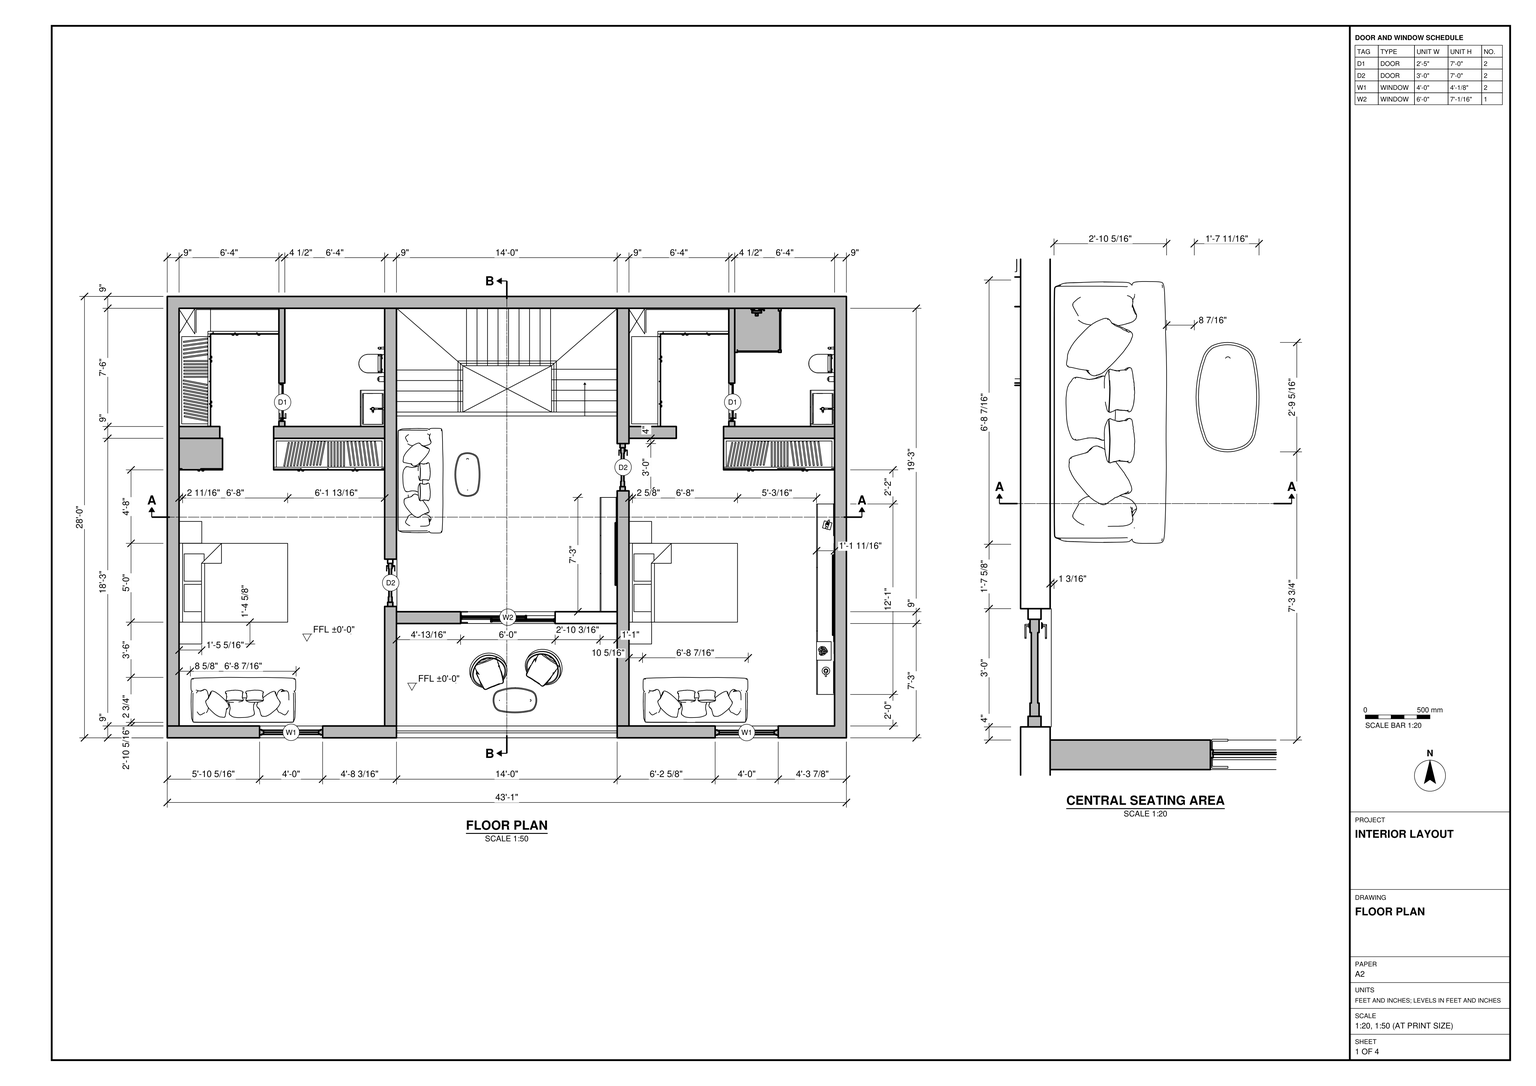
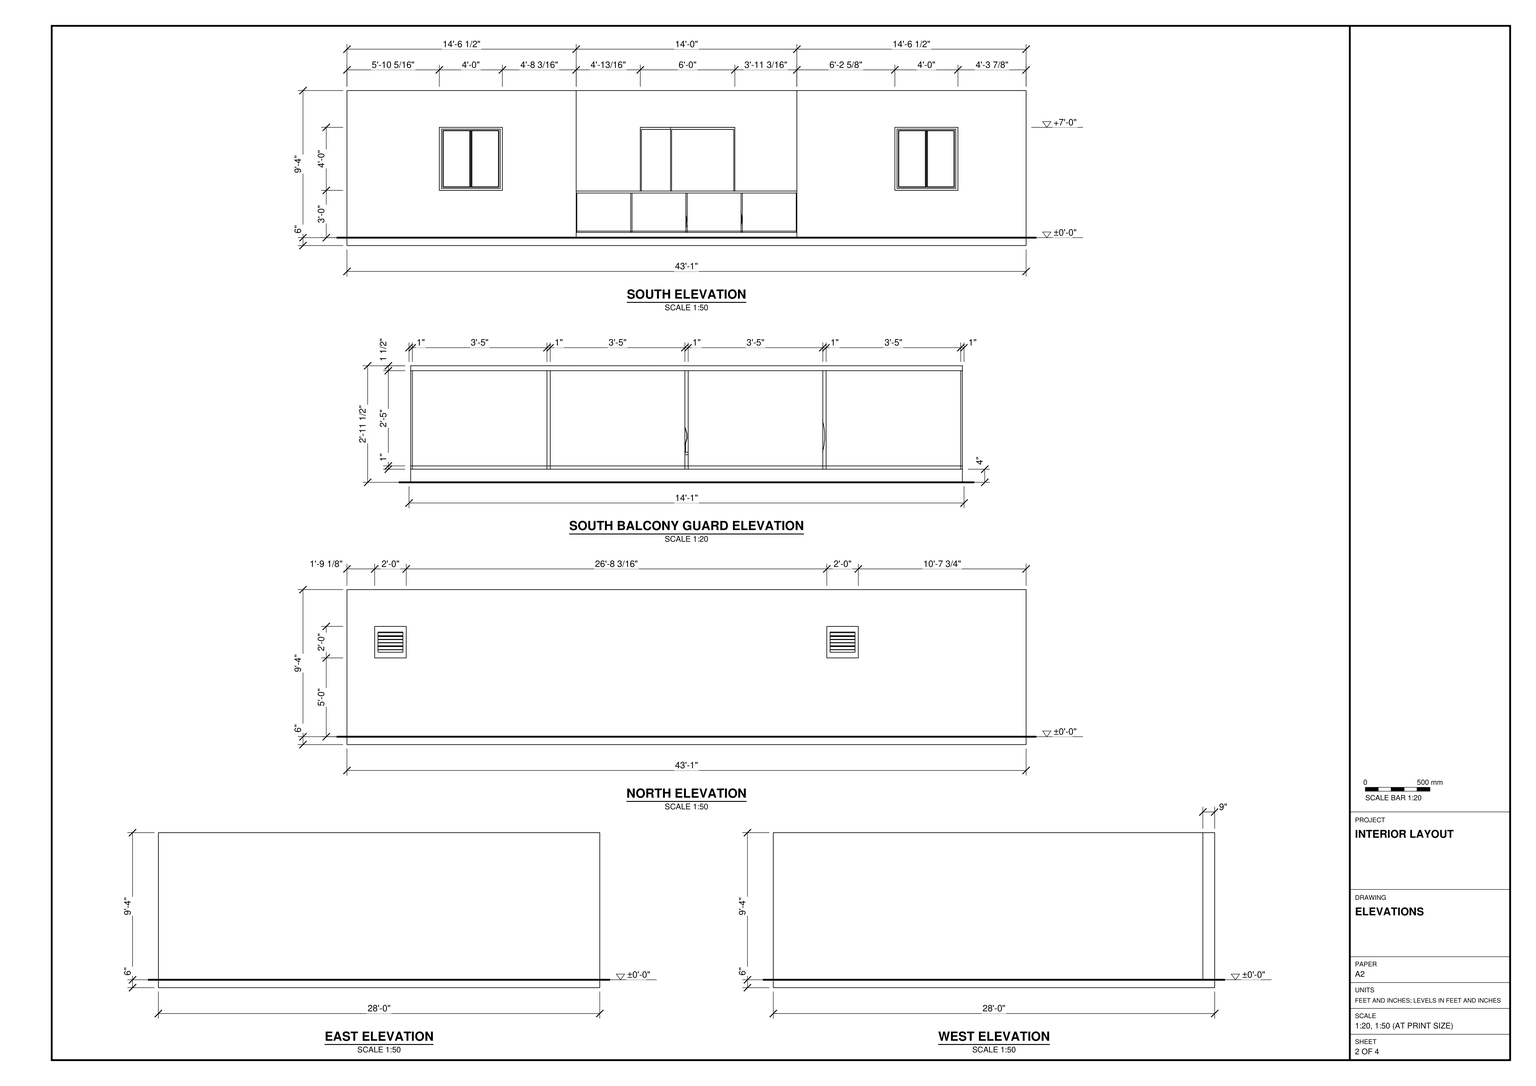
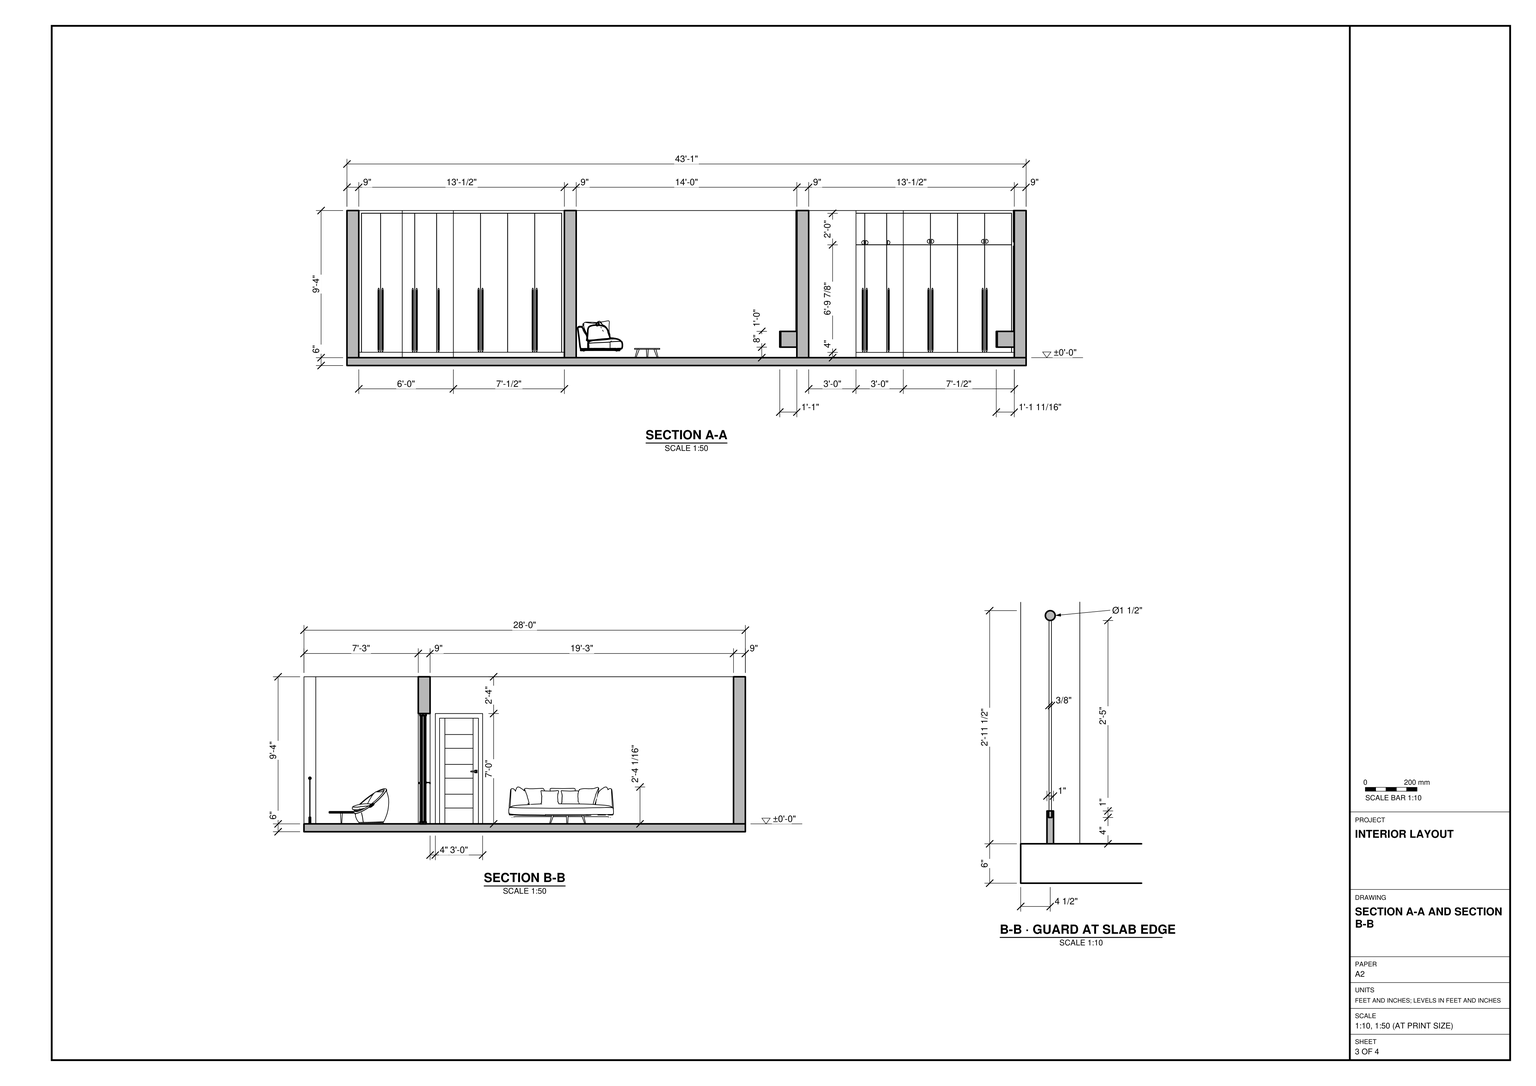
Build the single-storey interior in SketchUp from task_files/diagram_01.pdf. Work in feet and inches. Set the finished floor level to ±0'-0". The model measures 43'-1" east to west, 28'-0" north to south and 9'-10" from the underside of the slab to the top of the walls. Model the 6" floor slab, the 9" perimeter and main dividing walls, and the 4 1/2" partitions shown on the plan.

Lay out the two bedroom suites on either side of the 14'-0" central bay. In each suite, place the bed and sofa as drawn, fit the wardrobe and storage units along the indicated wall runs, and model the dressing area and adjoining bathroom with its fixtures. In the central bay, model the stair at the north end and the sitting area with the sofa, low table and facing wall unit. Recess the balcony between the bedrooms at the south end. Include its pair of chairs, table and panelled guard at the slab edge.

Fit the doors and window units to the scheduled openings. Use the elevations to locate the bedroom windows, the wider glazed opening facing the balcony and the louvred openings on the north wall. Keep shell elements and each furniture or joinery piece in separate groups or components, and use components for repeated parts. Decor and loose items may be any suitable library components, for example from 3D Warehouse. Save one SketchUp model as output_files/two_bedroom_suites_with_central_lounge_and_balcony.skp.

# SketchUp Ruby script. Lengths in inches.
U = 1.inch
M = Sketchup.active_model
def pt(a) = Geom::Point3d.new(a.map { |v| v * U })
def face(e, loops, mat)
  f = e.add_face(loops[0].map { |a| pt(a) })
  loops[1..].each { |l| e.add_face(l.map { |a| pt(a) }).erase! }
  f.material = f.back_material = mat if mat
  f
end
# faces: each face lists its corners as indices into pts; further lists are holes
def faces(e, pts, list, mat = nil) = list.each { |f| face(e, (f[0].is_a?(Array) ? f : [f]).map { |l| l.map { |i| pts[i] } }, mat) }
# xy, xz, yz: faces in a plane at the given z, y or x. An outline is a flat list of corners, or four numbers for a rectangle; further outlines are holes
def ring(l) = l.size == 4 ? [[l[0], l[1]], [l[2], l[1]], [l[2], l[3]], [l[0], l[3]]] : l.each_slice(2).to_a
def flat(e, list, mat, &to3) = list.each { |f| face(e, (f[0].is_a?(Array) ? f : [f]).map { |l| ring(l).map { |u, v| to3.(u, v) } }, mat) }
def xy(e, z, list, mat = nil) = flat(e, list, mat) { |x, y| [x, y, z] }
def xz(e, y, list, mat = nil) = flat(e, list, mat) { |x, z| [x, y, z] }
def yz(e, x, list, mat = nil) = flat(e, list, mat) { |y, z| [x, y, z] }
def lines(e, pts, list) = list.each { |a, b| e.add_line(pt(pts[a]), pt(pts[b])) }
# prism: a flat outline (further loops are holes) pulled along v
def prism(e, loops, v, mat = nil)
  f = face(e, loops, mat); d = Geom::Vector3d.new(v.map { |x| x * U })
  f.pushpull(f.normal.samedirection?(d) ? d.length : -d.length)
end
def box(e, o, s, mat = nil) = prism(e, [[o, [o[0] + s[0], o[1], o[2]], [o[0] + s[0], o[1] + s[1], o[2]], [o[0], o[1] + s[1], o[2]]]], [0, 0, s[2]], mat)
def at(x, y, z, deg = 0) = Geom::Transformation.translation(pt([x, y, z])) * Geom::Transformation.rotation(ORIGIN, Z_AXIS, deg.degrees)
def axes(o, x, y, z) = Geom::Transformation.new([*x, 0, *y, 0, *z, 0, *pt(o).to_a, 1])
def part(name) = M.definitions.add(name)
# library, detail: a bought-in or finely detailed component or shape, given as its bounding box
def library(name, o, s) = part(name).tap { |d| box(d.entities, o, s) }
def detail(e, o, s) = box(e.add_group.entities, o, s)
def put(e, d, t, mat = nil) = e.add_instance(d, t).tap { |i| i.material = mat if mat }
def group(e, t, mat = nil) = e.add_group.tap { |g| g.transformation = t; g.material = mat if mat }.entities
root = M.entities
M.materials.add("0207 AP 9584 Fervent Fuchsia-N").color = [176, 89, 135]
M.materials.add("0210 AP 9427 DELICATE PINK").color = [242, 226, 232]
M.materials.add("Glass Railing Color").color = [198, 198, 198]
M.materials.add("Railing Glass").color = [63, 150, 137]
M.materials["Railing Glass"].alpha = 0.13
M.materials.add("TEAKcrown-cut").color = [186, 122, 55]
M.materials.add("[Color M09]").color = [0, 0, 0]
M.materials.add("[Translucent Glass Gray]").color = [128, 128, 128]
M.materials["[Translucent Glass Gray]"].alpha = 0.5
M.materials.add("[Translucent_Glass_Gray]3").color = [255, 255, 255]
M.materials["[Translucent_Glass_Gray]3"].alpha = 0.5
M.materials.add("[Wood Floor]").color = [155, 105, 61]
M.materials.add("[Wood Veneer 02]").color = [190, 128, 91]
M.materials.add("dssd").color = [209, 209, 208]
c1 = library("Sliding windows",[317.26,-0.89,0.35],[175.04,8.85,122.84])
c2 = part("window full")
xy(c2.entities,0,[[0,0,14.17,66.54]])
xy(c2.entities,2.26,[[12.2,2.26,14.17,64.28]],"[Wood Floor]")
xy(c2.entities,2.36,[[0,2.36,1.97,64.17]],"[Wood Floor]")
xy(c2.entities,3.74,[[11.42,3.74,12.2,32.875],[11.42,33.66,12.2,62.79]],"[Wood Floor]")
xy(c2.entities,3.9375,[[1.97,3.9375,2.76,32.77],[1.97,33.76,2.76,62.6]],"[Wood Floor]")
xy(c2.entities,4.18,[[2.76,4.18,7.09,32.09],[7.09,4.18,11.42,32.09],[2.76,34.45,7.09,62.35],[7.09,34.45,11.42,62.35]],"[Wood Floor]")
xy(c2.entities,69.83,[[2.76,4.18,7.09,32.09],[7.09,32.09,11.42,34.45],[2.76,34.45,7.09,62.35]])
xy(c2.entities,69.83,[[7.09,4.18,11.42,32.09],[7.09,34.45,11.42,62.35]],"[Wood Floor]")
xy(c2.entities,70.08,[[1.97,3.9375,2.76,32.77],[1.97,33.76,2.76,62.6]])
xy(c2.entities,70.27,[[11.42,32.875,12.2,33.66]])
xy(c2.entities,70.27,[[11.42,3.74,12.2,32.875],[11.42,33.66,12.2,62.79]],"[Wood Floor]")
xy(c2.entities,71.65,[[0,2.36,1.97,64.17]])
xy(c2.entities,71.76,[[12.2,2.26,14.17,64.28]],"[Wood Floor]")
xy(c2.entities,74.02,[[0,0,14.17,66.54]],"[Wood Floor]")
xz(c2.entities,0,[[0,0,14.17,74.02]],"[Wood Floor]")
xz(c2.entities,2.26,[[12.2,2.26,14.17,71.76]],"[Wood Floor]")
xz(c2.entities,2.36,[[0,2.36,1.97,71.65]],"[Wood Floor]")
xz(c2.entities,3.74,[[11.42,3.74,12.2,70.27]],"[Wood Floor]")
xz(c2.entities,3.9375,[[1.97,3.9375,2.76,70.08]],"[Wood Floor]")
xz(c2.entities,4.18,[[2.76,4.18,7.09,69.83],[7.09,4.18,11.42,69.83]],"[Wood Floor]")
xz(c2.entities,32.09,[[2.76,4.18,11.42,69.83]],"[Wood Floor]")
xz(c2.entities,32.77,[[1.97,3.9375,2.76,70.08]],"[Wood Floor]")
xz(c2.entities,32.875,[[11.42,3.74,12.2,70.27]],"[Wood Floor]")
xz(c2.entities,33.66,[[11.42,3.74,12.2,47.88],[11.42,47.88,12.2,70.27]],"[Wood Floor]")
xz(c2.entities,33.76,[[1.97,3.9375,2.76,70.08]],"[Wood Floor]")
xz(c2.entities,34.45,[[2.76,4.18,11.42,69.83]],"[Wood Floor]")
xz(c2.entities,62.35,[[2.76,4.18,7.09,69.83],[7.09,4.18,11.42,69.83]],"[Wood Floor]")
xz(c2.entities,62.6,[[1.97,3.9375,2.76,70.08]],"[Wood Floor]")
xz(c2.entities,62.79,[[11.42,3.74,12.2,70.27]],"[Wood Floor]")
xz(c2.entities,64.17,[[0,2.36,1.97,71.65]],"[Wood Floor]")
xz(c2.entities,64.28,[[12.2,2.26,14.17,71.76]],"[Wood Floor]")
xz(c2.entities,66.54,[[0,0,14.17,74.02]],"[Wood Floor]")
yz(c2.entities,0,[[[0,0,66.54,74.02],[2.36,2.36,64.17,71.65]]],"[Wood Floor]")
yz(c2.entities,1.97,[[[2.36,2.36,64.17,71.65],[33.76,3.9375,62.6,70.08],[3.9375,3.9375,32.77,70.08]]],"[Wood Floor]")
yz(c2.entities,2.76,[[32.77,3.9375,33.76,4.18],[32.77,4.18,33.76,69.83],[32.77,69.83,33.76,70.08]])
yz(c2.entities,2.76,[[[3.9375,3.9375,32.77,70.08],[4.18,4.18,32.09,69.83]],[[33.76,3.9375,62.6,70.08],[34.45,4.18,62.35,69.83]]],"[Wood Floor]")
yz(c2.entities,7.09,[[4.18,4.18,62.35,69.83]],"[Translucent Glass Gray]")
yz(c2.entities,11.42,[[32.875,69.83,33.66,70.27]])
yz(c2.entities,11.42,[[[3.74,3.74,32.875,70.27],[4.18,4.18,32.09,69.83]],[[33.66,3.74,62.79,70.27],[34.45,4.18,62.35,69.83]]],"[Wood Floor]")
yz(c2.entities,12.2,[[[2.26,2.26,64.28,71.76],[33.66,3.74,62.79,70.27],[3.74,3.74,32.875,70.27]]],"[Wood Floor]")
yz(c2.entities,14.17,[[[0,0,66.54,74.02],[2.26,2.26,64.28,71.76]]],"[Wood Floor]")
p = [[11.42,32.875,70.27],[11.42,32.875,70.28]]
lines(c2.entities,p,[[0,1]])
c3 = part("Component\#10")
box(c3.entities,[0,0,0],[19,0.25,3.7],"[Translucent_Glass_Gray]3")
c4 = part("Ventilation_window")
g1 = group(c4.entities,at(-76.91,6.38,0),"TEAKcrown-cut")
xy(g1,-1.7,[[0,0,24,3]])
xy(g1,2.5,[[2.5,0,21.5,3]])
xy(g1,17.5,[[2.5,0,21.5,3]])
xy(g1,21.7,[[0,0,24,3]])
xz(g1,0,[[[0,-1.7,24,21.7],[2.5,2.5,21.5,17.5]]],"TEAKcrown-cut")
xz(g1,3,[[[0,-1.7,24,21.7],[2.5,2.5,21.5,17.5]]])
yz(g1,0,[[0,-1.7,3,21.7]])
yz(g1,2.5,[[0,2.5,3,2.5,3,4.31,0,6.48],[3,4.31,3,17.5,0,17.5,0,6.48]])
yz(g1,21.5,[[0,2.5,3,17.5]])
yz(g1,24,[[0,-1.7,3,21.7]])
put(g1,c3,axes([2.5,3.14,11.94],[1,0,0],[0,0.58779,0.80902],[0,-0.80902,0.58779]))
put(g1,c3,axes([2.5,3.16,14.6],[1,0,0],[0,0.58779,0.80902],[0,-0.80902,0.58779]))
put(g1,c3,axes([2.5,3,4.31],[1,0,0],[0,0.58779,0.80902],[0,-0.80902,0.58779]))
put(g1,c3,axes([2.5,3.14,9.46],[1,0,0],[0,0.58779,0.80902],[0,-0.80902,0.58779]))
put(g1,c3,axes([2.5,2.99,7.08],[1,0,0],[0,0.58779,0.80902],[0,-0.80902,0.58779]))
c5 = library("door by lz",[5.91,-4.92,0],[35.43,6.61,78.74])
c6 = library("3D DOOR",[-0.52,0,0],[35.44,5.29,86.61])
c7 = library("LXS-WHT-67903",[-6.02,-15.85,-9.41],[15.75,23.61,5.61])
c8 = library("Wall-hung toilet",[0,0,0],[28.35,19.69,42.125])
c9 = library("Shower set",[0,0,0],[23.15,11.69,55.71])
c10 = library("3-ROBINET CLC2",[-0.79,-7.28,0],[1.58,8.07,7.48])
c11 = library("11-POIGNEE CLC2",[-0.59,-0.59,0],[1.18,1.18,1.22])
c12 = library("Balcony_Chair_9942",[0,-48.42,0],[44.51,48.42,45.43])
c13 = library("sofaD71839)",[0.35,-39.08,0.31],[80.46,34.29,30.24])
c14 = part("200mm Half Round Handle")
xz(c14.entities,0,[[3.9375,0,3.9375,7.875,3.42,7.84,2.92,7.74,2.43,7.57,1.97,7.35,1.54,7.06,1.15,6.72,0.8125,6.33,0.53,5.91,0.3,5.44,0.13,4.96,0.03,4.45,0,3.9375,0.03,3.42,0.13,2.92,0.3,2.43,0.53,1.97,0.8125,1.54,1.15,1.15,1.54,0.8125,1.97,0.53,2.43,0.3,2.92,0.13,3.42,0.03]],"[Color M09]")
xz(c14.entities,0.12,[[3.82,0.01,3.42,0.03,2.92,0.13,2.43,0.3,1.97,0.53,1.54,0.8125,1.15,1.15,0.8125,1.54,0.53,1.97,0.3,2.43,0.13,2.92,0.03,3.42,0,3.9375,0.03,4.45,0.13,4.96,0.3,5.44,0.53,5.91,0.8125,6.33,1.15,6.72,1.54,7.06,1.97,7.35,2.43,7.57,2.92,7.74,3.42,7.84,3.82,7.87]],"[Color M09]")
xz(c14.entities,0.91,[[3.9375,0,3.82,0.01,3.82,7.87,3.9375,7.875]],"[Color M09]")
yz(c14.entities,3.82,[[0.12,0.01,0.91,7.87]],"[Color M09]")
yz(c14.entities,3.9375,[[0,0,0.91,7.875]],"[Color M09]")
p = [[3.42,0,0.03],[2.92,0,0.13],[2.92,0.12,0.13],[3.42,0.12,0.03],[3.9375,0,0],[3.82,0.12,0.01],
  [3.82,0.91,0.01],[3.9375,0.91,0],[2.43,0,0.3],[2.43,0.12,0.3],[1.97,0,0.53],[1.97,0.12,0.53],
  [1.54,0,0.8125],[1.54,0.12,0.8125],[1.15,0,1.15],[1.15,0.12,1.15],[0.8125,0,1.54],[0.8125,0.12,1.54],
  [0.53,0,1.97],[0.53,0.12,1.97],[0.3,0,2.43],[0.3,0.12,2.43],[0.13,0,2.92],[0.13,0.12,2.92],
  [0.03,0,3.42],[0.03,0.12,3.42],[0,0,3.9375],[0,0.12,3.9375],[0.03,0,4.45],[0.03,0.12,4.45],
  [0.13,0,4.96],[0.13,0.12,4.96],[0.3,0,5.44],[0.3,0.12,5.44],[0.53,0,5.91],[0.53,0.12,5.91],
  [0.8125,0,6.33],[0.8125,0.12,6.33],[1.15,0,6.72],[1.15,0.12,6.72],[1.54,0,7.06],[1.54,0.12,7.06],
  [1.97,0,7.35],[1.97,0.12,7.35],[2.43,0,7.57],[2.43,0.12,7.57],[2.92,0,7.74],[2.92,0.12,7.74],
  [3.42,0,7.84],[3.42,0.12,7.84],[3.9375,0,7.875],[3.9375,0.91,7.875],[3.82,0.91,7.87],[3.82,0.12,7.87]]
faces(c14.entities,p,[[0,1,2,3],[4,0,3,5,6,7],[1,8,9,2],[8,10,11,9],[10,12,13,11],[12,14,15,13],[14,16,17,15],[16,18,19,17],
  [18,20,21,19],[20,22,23,21],[22,24,25,23],[24,26,27,25],[26,28,29,27],[28,30,31,29],[30,32,33,31],[32,34,35,33],
  [34,36,37,35],[36,38,39,37],[38,40,41,39],[40,42,43,41],[42,44,45,43],[44,46,47,45],[46,48,49,47],[48,50,51,52,53,49]],"[Color M09]")
c15 = library("Drawing1 INTERNSHIP1.dwg",[0,76.08,-3.29],[517,336,23.29])
c16 = part("Group11\#1")
xy(c16.entities,0,[[0,76.08,0,412.08,517,412.08,517,76.08,342.5,76.08,342.5,85.08,508,85.08,508,403.08,9,403.08,9,85.08,174.5,85.08,174.5,76.08],[174.5,76.08,342.5,85.08]])
xy(c16.entities,36,[[417.1,76.08,465.1,85.08]])
xy(c16.entities,60,[[127.73,403.08,151.73,412.08],[471.9,403.08,495.9,412.08]])
xy(c16.entities,84,[[417.1,76.08,465.1,85.08],[127.73,403.08,151.73,412.08],[471.9,403.08,495.9,412.08]])
xy(c16.entities,112,[[0,76.08,9,76.08,9,403.08,508,403.08,508,85.08,342.5,85.08,342.5,76.08,517,76.08,517,412.08,0,412.08]])
xz(c16.entities,76.08,[[[342.5,0,517,112],[417.1,36,465.1,84]]])
xz(c16.entities,85.08,[[[342.5,0,508,112],[417.1,36,465.1,84]]])
xz(c16.entities,403.08,[[[9,0,508,112],[471.9,60,495.9,84],[127.73,60,151.73,84]]])
xz(c16.entities,412.08,[[[0,0,517,112],[471.9,60,495.9,84],[127.73,60,151.73,84]]])
yz(c16.entities,0,[[76.08,0,412.08,112]])
yz(c16.entities,9,[[85.08,0,403.08,112]])
yz(c16.entities,127.73,[[403.08,60,412.08,84]])
yz(c16.entities,151.73,[[403.08,60,412.08,84]])
yz(c16.entities,342.5,[[76.08,0,85.08,112]])
yz(c16.entities,417.1,[[76.08,36,85.08,84]])
yz(c16.entities,465.1,[[76.08,36,85.08,84]])
yz(c16.entities,471.9,[[403.08,60,412.08,84]])
yz(c16.entities,495.9,[[403.08,60,412.08,84]])
yz(c16.entities,508,[[85.08,0,403.08,112]])
yz(c16.entities,517,[[76.08,0,412.08,112]])
c17 = part("Group12\#1")
prism(c17.entities,[[[174.5,85.08,0],[174.5,176.08,0],[174.5,176.08,84],[174.5,212.08,84],[174.5,212.08,0],[174.5,403.08,0],[174.5,403.08,112],[174.5,85.08,112]]],[-9,0,0])
c18 = library("Group359\#1",[-14.875,-46,0],[29.75,92,0.47])
c19 = part("Group13\#1")
xy(c19.entities,0,[[342.5,85.08,342.48,264.08,351.48,264.08,351.5,85.08],[342.48,300.08,342.47,403.08,351.47,403.08,351.48,300.08]])
xy(c19.entities,84,[[342.48,264.08,351.48,300.08]])
xy(c19.entities,112,[[342.5,85.08,351.5,85.08,351.47,403.08,342.47,403.08,342.48,259.08,342.49,174.45,342.49,172.08],[342.49,174.45,342.48,259.08,342.48,229.33]])
xz(c19.entities,85.08,[[342.5,0,351.5,112]])
xz(c19.entities,264.08,[[342.48,0,351.48,84]])
xz(c19.entities,300.08,[[342.48,0,351.48,84]])
xz(c19.entities,403.08,[[342.47,0,351.47,112]])
yz(c19.entities,342.48,[[229.33,20,259.08,112]])
p = [[342.47,403.08,0],[342.48,300.08,0],[342.48,300.08,84],[342.48,264.08,84],[342.48,264.08,0],[342.5,85.08,0],
  [342.5,85.08,112],[342.49,172.08,112],[342.49,174.45,112],[342.48,259.08,112],[342.47,403.08,112],[351.5,85.08,0],
  [351.48,264.08,0],[351.48,264.08,84],[351.48,300.08,84],[351.48,300.08,0],[351.47,403.08,0],[351.47,403.08,112],
  [351.5,85.08,112],[342.48,229.33,20],[342.49,172.08,20],[342.48,229.33,112]]
faces(c19.entities,p,[[0,1,2,3,4,5,6,7,8,9,10],[11,12,13,14,15,16,17,18],[19,20,7,8,21]])
put(c19.entities,c18,axes([342.48,244.21,66],[0,-1,0],[0,0,1],[-1,0,0]),"[Wood Veneer 02]")
c20 = part("Group14\#1")
prism(c20.entities,[[[342.49,172.08,0],[295.29,172.08,0],[295.29,172.08,84],[223.29,172.08,84],[223.29,172.08,0],[174.5,172.08,0],[174.5,172.08,112],[342.49,172.08,112]]],[0,-9,0])
c21 = part("Group15\#1")
box(c21.entities,[9,304.08,0],[31,9,112])
c22 = part("Group16\#1")
box(c22.entities,[81,304.08,0],[84.5,9,112])
c23 = part("Group17\#1")
box(c23.entities,[351.5,304.08,0],[36,9,112])
c24 = part("Group18\#1")
box(c24.entities,[423.5,304.08,0],[84.5,9,112])
c25 = part("Group20\#1")
prism(c25.entities,[[[89.5,313.08,0],[89.5,317.08,0],[89.5,317.08,84],[89.5,346.08,84],[89.5,346.08,0],[89.5,403.08,0],[89.5,403.08,112],[89.5,313.08,112]]],[-4.5,0,0])
p = [[427.5,346,0.08],[432,346,0.08]]
lines(c25.entities,p,[[0,1]])
c26 = part("Group21\#1")
prism(c26.entities,[[[432,313.08,0],[432,317.08,0],[432,317.08,84],[432,346.08,84],[432,346.08,0],[432,403.08,0],[432,403.08,112],[432,313.08,112]]],[-4.5,0,0])
c27 = part("Group77\#1")
prism(c27.entities,[[[0,85.08,0],[0,85.08,112],[174.5,85.08,112],[174.5,85.08,0]],[[70.29,85.08,36],[118.29,85.08,36],[118.29,85.08,84],[70.29,85.08,84]]],[0,-9,0])
c28 = library("Group\#6",[0,0,0],[75.97,90,112])
c29 = part("Glass Rail Spacer")
box(c29.entities,[-0.5,-0.25,0],[1,0.5,1],"Glass Railing Color")
c30 = part("Group112\#1")
prism(c30.entities,[[[0.54,0,1.27],[0.38,0,1.39],[0.21,0,1.47],[0.01,0,1.5],[-0.18,0,1.48],[-0.37,0,1.41],[-0.52,0,1.29],[-0.64,0,1.13],[-0.72,0,0.96],[-0.75,0,0.76],[-0.73,0,0.57],[-0.66,0,0.38],[-0.54,0,0.23],[-0.38,0,0.11],[-0.21,0,0.03],[-0.01,0,0],[0.18,0,0.02],[0.37,0,0.09],[0.52,0,0.21],[0.64,0,0.37],[0.72,0,0.54],[0.75,0,0.74],[0.73,0,0.93],[0.66,0,1.12]]],[0,169,0],"[Color M09]")
c31 = part("Group115\#1")
xy(c31.entities,0,[[-0.5,0,0.5,169]],"Glass Railing Color")
xy(c31.entities,4,[[-0.25,0,0.25,169]],"Glass Railing Color")
xy(c31.entities,5,[[-0.5,0,-0.25,169],[0.25,0,0.5,169]],"[Color M09]")
xz(c31.entities,0,[[-0.5,0,0.5,0,0.5,5,0.25,5,0.25,4,-0.25,4,-0.25,5,-0.5,5]],"Glass Railing Color")
xz(c31.entities,169,[[-0.5,0,-0.5,5,-0.25,5,-0.25,4,0.25,4,0.25,5,0.5,5,0.5,0]],"Glass Railing Color")
yz(c31.entities,-0.5,[[0,0,169,5]],"[Color M09]")
yz(c31.entities,-0.25,[[0,4,169,5]],"Glass Railing Color")
yz(c31.entities,0.25,[[0,4,169,5]],"Glass Railing Color")
yz(c31.entities,0.5,[[0,0,169,5]],"[Color M09]")
c32 = part("Group116\#1")
box(c32.entities,[-0.1875,0,0],[0.375,41,30],"Railing Glass")
c33 = part("Group117\#1")
box(c33.entities,[-0.1875,0,0],[0.375,41,30],"Railing Glass")
c34 = part("Group118\#1")
box(c34.entities,[-0.1875,0,0],[0.375,41,30],"Railing Glass")
c35 = part("Group119\#1")
box(c35.entities,[-0.1875,0,0],[0.375,41,30],"Railing Glass")
c36 = part("Glass Railing")
put(c36.entities,c29,at(0,0,4))
put(c36.entities,c29,at(42,0,4))
put(c36.entities,c29,at(84,0,4))
put(c36.entities,c29,at(126,0,4))
put(c36.entities,c29,at(168,0,4))
put(c36.entities,c30,at(-0.5,0,34,-90),"Glass Railing Color")
put(c36.entities,c31,at(-0.5,0,0,-90),"Glass Railing Color")
put(c36.entities,c32,at(0.5,0,4,-90),"Railing Glass")
put(c36.entities,c33,at(42.5,0,4,-90),"Railing Glass")
put(c36.entities,c34,at(84.5,0,4,-90),"Railing Glass")
put(c36.entities,c35,at(126.5,0,4,-90),"Railing Glass")
c37 = part("Group\#346")
detail(c37.entities,[0,0,0],[11.18,0.75,1.1])
c38 = library("Group\#15",[-0.24,0,0],[0.48,145.01,92])
c39 = part("Obj3d66-852568-53-874_002_Defintion")
xz(c39.entities,385.75,[[-1015.78,-10.2,-1015.78,10.2,-515.78,10.2],[-1015.78,-10.2,-515.78,10.2,-515.78,-10.2],[-15.78,-10.2,-515.78,10.2,-15.78,10.2],[-515.78,-10.2,-515.78,10.2,-15.78,-10.2]],"dssd")
yz(c39.entities,-1015.78,[[-379.41,-49.47,-393.27,-30.41,-189.45,-30.41],[-379.41,-49.47,-189.45,-30.41,-181.19,-49.47],[-181.19,-49.47,-189.45,-30.41,388.11,-30.41],[-181.19,-49.47,388.11,-30.41,393.73,-49.47],[-393.27,-30.41,-400.42,-10.2,-193.44,-10.2],
  [-393.27,-30.41,-193.44,-10.2,-189.45,-30.41],[-189.45,-30.41,-193.44,-10.2,385.75,-10.2],[-189.45,-30.41,385.75,-10.2,388.11,-30.41],[-400.42,-10.2,-193.44,10.2,-193.44,-10.2],[-400.42,-10.2,-400.42,10.2,-193.44,10.2],
  [-193.44,-10.2,-193.44,10.2,385.75,10.2],[-193.44,-10.2,385.75,10.2,385.75,-10.2],[-400.42,10.2,-393.27,30.41,-193.44,10.2],[-193.44,10.2,-393.27,30.41,-189.45,30.41],[-193.44,10.2,-189.45,30.41,385.75,10.2],
  [385.75,10.2,-189.45,30.41,388.11,30.41],[-393.27,30.41,-379.41,49.47,-189.45,30.41],[-189.45,30.41,-379.41,49.47,-181.19,49.47],[-189.45,30.41,-181.19,49.47,388.11,30.41],[388.11,30.41,-181.19,49.47,393.73,49.47]],"dssd")
yz(c39.entities,-15.78,[[-379.41,-49.47,-189.45,-30.41,-393.27,-30.41],[-379.41,-49.47,-181.19,-49.47,-189.45,-30.41],[-181.19,-49.47,388.11,-30.41,-189.45,-30.41],[-181.19,-49.47,393.74,-49.47,388.11,-30.41],[-393.27,-30.41,-193.44,-10.2,-400.42,-10.2],
  [-393.27,-30.41,-189.45,-30.41,-193.44,-10.2],[-189.45,-30.41,385.75,-10.2,-193.44,-10.2],[-189.45,-30.41,388.11,-30.41,385.75,-10.2],[-193.44,-10.2,-193.44,10.2,-400.42,10.2],[-400.42,-10.2,-193.44,-10.2,-400.42,10.2],
  [-193.44,-10.2,385.75,-10.2,385.75,10.2],[-193.44,-10.2,385.75,10.2,-193.44,10.2],[-400.42,10.2,-193.44,10.2,-393.27,30.41],[-193.44,10.2,-189.45,30.41,-393.27,30.41],[-193.44,10.2,385.75,10.2,-189.45,30.41],
  [385.75,10.2,388.11,30.41,-189.45,30.41],[-393.27,30.41,-189.45,30.41,-379.41,49.47],[-189.45,30.41,-181.19,49.47,-379.41,49.47],[-189.45,30.41,388.11,30.41,-181.19,49.47],[388.11,30.41,393.73,49.47,-181.19,49.47]],"dssd")
p = [[-515.78,388.11,-30.41],[-515.78,393.74,-49.47],[-1015.78,393.73,-49.47],[-1015.78,388.11,-30.41],[-15.78,388.11,-30.41],[-15.78,393.74,-49.47],
  [-515.78,385.75,-10.2],[-1015.78,385.75,-10.2],[-15.78,385.75,-10.2],[-515.78,388.11,30.41],[-515.78,385.75,10.2],[-1015.78,385.75,10.2],
  [-1015.78,388.11,30.41],[-15.78,388.11,30.41],[-15.78,385.75,10.2],[-515.78,393.74,49.47],[-1015.78,393.73,49.47],[-15.78,393.73,49.47]]
faces(c39.entities,p,[[0,1,2],[2,3,0],[0,4,5],[5,1,0],[6,0,3],[3,7,6],[6,8,4],[4,0,6],
  [9,10,11],[11,12,9],[9,13,14],[14,10,9],[15,9,12],[12,16,15],[15,17,13],[13,9,15]],"dssd")
c40 = library("Group131",[13.13,-6.23,10.37],[4.44,3.5,0.46])
c41 = library("Group95",[3.61,-3.27,10.38],[1.32,1.2,0.77])
c42 = library("Group94",[3.24,-2.96,11.13],[1.71,0.46,6.32])
c43 = library("Group74",[13.16,-2.77,10.375],[2.82,2.4,6.94])
c44 = library("Group76",[14.28,-5.9,10.43],[2.93,2.9,2.07])
put(root,c1,axes([92.79,88.28,-0.32],[0.41134,0,0],[0,1,0],[0,0,0.68449]))
put(root,c2,axes([417.1,5.95,36],[0,-0.273,0],[0.72142,0,0],[0,0,0.65]))
put(root,c2,axes([70.29,6.125,36],[0,-0.273,0],[0.72142,0,0],[0,0,0.65]))
put(root,c4,axes([204.64,319.57,61.74],[1,0,0],[0,1.4715,0],[0,0,1.02564]))
put(root,c4,axes([548.8125,319.57,61.74],[1,0,0],[0,1.4715,0],[0,0,1.02564]))
put(root,c5,axes([171.72,142.01,0],[0,-1.016,0],[1,0,0],[0,0,1.0668]))
put(root,c5,axes([348.625,230.01,0],[0,-1.016,0],[1,0,0],[0,0,1.0668]))
put(root,c6,axes([433.08,241.42,0],[0,0.81844,0],[-1,0,0],[0,0,0.96982]))
put(root,c6,axes([90.46,241.42,0],[0,0.81844,0],[-1,0,0],[0,0,0.96982]))
put(root,c7,at(154.65,254.42,37.05))
put(root,c8,at(165.5,270.72,0,90))
put(root,c9,at(443.97,327,34.29,-90))
put(root,c7,at(497.15,254.42,37.05))
put(root,c8,at(508,270.72,0,90))
put(root,c10,at(164.71,250.49,32.56,-90))
put(root,c10,at(507.21,250.49,32.56,-90))
put(root,c11,axes([434.77,293.88,54.09],[1,0,0],[0,0,1],[0,-1,0]))
put(root,c12,axes([267.49,51.04,0],[0.32992,0.48913,0],[-0.48913,0.32992,0],[0,0,0.59]))
put(root,c12,axes([235.48,34.02,0],[-0.20469,0.55335,0],[-0.55335,-0.20469,0],[0,0,0.59]))
put(root,c13,at(170.88,155.27,-0.31,90))
put(root,c14,axes([446.74,203.59,90.15],[-0.46,0,0],[0,0.46,0],[0,0,-0.4094]))
put(root,c14,axes([441.74,203.59,90.15],[0.46,0,0],[0,0.46,0],[0,0,-0.4094]))
put(root,c14,axes([488.11,203.59,90.15],[-0.46,0,0],[0,0.46,0],[0,0,-0.4094]))
put(root,c14,axes([482.99,203.59,90.15],[0.46,0,0],[0,0.46,0],[0,0,-0.4094]))
put(root,c14,axes([375.91,256.61,89.82],[0,-0.46,0],[-0.46,0,0],[0,0,-0.4094]))
put(root,c14,axes([375.91,251.8,89.82],[0,0.46,0],[-0.46,0,0],[0,0,-0.4094]))
put(root,c14,axes([375.91,286.03,89.82],[0,0.46,0],[-0.46,0,0],[0,0,-0.4094]))
put(root,c14,axes([375.91,290.84,89.82],[0,-0.46,0],[-0.46,0,0],[0,0,-0.4094]))
put(root,c14,axes([391.87,307.05,89.22],[0.46,0,0],[0,0.46,0],[0,0,-0.4094]))
put(root,c14,axes([396.68,307.05,89.22],[-0.46,0,0],[0,0.46,0],[0,0,-0.4094]))
put(root,c14,axes([413.35,307.05,89.22],[-0.46,0,0],[0,0.46,0],[0,0,-0.4094]))
put(root,c15,at(0,-76.08,0))
put(root,c13,at(98.41,6.9375,-0.31,-180))
put(root,c13,at(442.6,6.9375,-0.31,-180))
put(root,c16,at(0,-76.08,0))
put(root,c17,at(0,-76.08,0))
put(root,c19,at(0,-76.08,0))
put(root,c20,at(0,-76.08,0))
put(root,c21,at(0,-76.08,0))
put(root,c22,at(0,-76.08,0))
put(root,c23,at(0,-76.08,0))
put(root,c24,at(0,-76.08,0))
put(root,c25,at(0,-76.08,0))
put(root,c26,at(0,-76.08,0))
g2 = group(root,at(0,0,-6))
box(g2,[0,0,0],[517,336,6])
g3 = group(root,at(146.93,237,0))
xy(g3,0,[[0.63,0,18.57,27.57]])
xy(g3,4,[[0,0,0.63,13.85],[0,13.85,0.63,14.79],[0,14.91,0.63,27.57]])
xy(g3,28,[[0,0,0.63,14.79],[0.63,0,18.57,27.57],[0,14.91,0.63,27.57]])
xz(g3,0,[[0.63,0,18.57,28],[0,4,0.63,28]])
xz(g3,14.79,[[0,4,0.63,28]])
xz(g3,14.91,[[0,4,0.63,28]])
xz(g3,27.57,[[0.63,0,18.57,28],[0,4,0.63,28]])
yz(g3,0,[[0,4,2,28],[2,4,2.12,28],[2.12,4,14.79,28],[14.91,4,27.57,28]])
yz(g3,0.63,[[0,0,27.57,4],[0,4,13.85,28],[13.85,4,14.79,28],[14.79,4,14.91,28],[14.91,4,27.57,28]])
yz(g3,18.57,[[0,0,27.57,28]])
p = [[0,14.85,4],[0.63,14.85,4]]
lines(g3,p,[[0,1]])
put(root,c27,at(0,-76.08,0))
g4 = group(root,at(423.5,204.01,0),"0210 AP 9427 DELICATE PINK")
xy(g4,0,[[0,2,84.5,23.96]])
xy(g4,4,[[20.74,0,20.74,0.71,0,0.71,0,2,84.5,2,84.5,0.71,82.38,0.71,82.38,0,61.99,0,61.99,0.71,41.25,0.71,41.25,0],[82.5,0,84.5,0.71]])
xy(g4,4,[[0,0,20.625,0.71],[41.37,0,61.875,0.71]],"0207 AP 9584 Fervent Fuchsia-N")
xy(g4,85.88,[[0,0,20.625,0.71],[20.74,0,41.25,0.71],[41.37,0,61.875,0.71],[61.99,0,82.38,0.71]],"0207 AP 9584 Fervent Fuchsia-N")
xy(g4,86,[[0,0,20.625,0.71],[20.74,0,41.25,0.71],[41.37,0,61.875,0.71],[61.99,0,82.38,0.71]])
xy(g4,109.88,[[0,0,20.625,0.71],[20.74,0,41.25,0.71],[41.37,0,61.875,0.71],[61.99,0,82.38,0.71]])
xy(g4,110,[[0,0,82.5,0.71]])
xy(g4,112,[[0,0,84.5,0.71],[0,0.71,84.5,23.96]])
xz(g4,0,[[82.5,4,84.5,4,84.5,112,0,112,0,110,82.5,110],[0,86,20.625,109.88],[20.74,86,41.25,109.88],[41.37,86,61.875,109.88],[61.99,86,82.38,109.88]])
xz(g4,0,[[0,4,20.625,85.88],[20.74,4,41.25,85.88],[41.37,4,61.875,85.88],[61.99,4,82.38,85.88]],"0207 AP 9584 Fervent Fuchsia-N")
xz(g4,0.71,[[82.5,4,82.5,110,0,110,0,112,84.5,112,84.5,4],[[20.625,4,20.74,4,20.74,85.88,41.25,85.88,41.25,4,41.37,4,41.37,85.88,61.875,85.88,61.875,4,61.99,4,61.99,85.88,82.38,85.88,82.38,4,82.5,4,82.5,110,0,110,0,109.88,20.625,109.88,20.625,86,0,86,0,85.88,20.625,85.88],[41.37,86,61.875,109.88],[20.74,86,41.25,109.88],[61.99,86,82.38,109.88]],[0,86,20.625,109.88]])
xz(g4,0.71,[[0,4,20.625,85.88],[41.37,4,61.875,85.88]],"0207 AP 9584 Fervent Fuchsia-N")
xz(g4,2,[[0,0,84.5,4]])
xz(g4,23.96,[[0,0,84.5,112]])
yz(g4,0,[[2,0,2,4,0.71,4,0.71,112,23.96,112,23.96,0],[0,86,0.71,109.88],[0,110,0.71,112]])
yz(g4,0,[[0,4,0.71,85.88]],"0207 AP 9584 Fervent Fuchsia-N")
yz(g4,20.625,[[0,86,0.71,109.88]])
yz(g4,20.625,[[0,4,0.71,85.88]],"0207 AP 9584 Fervent Fuchsia-N")
yz(g4,20.74,[[0,86,0.71,109.88]])
yz(g4,20.74,[[0,4,0.71,85.88]],"0207 AP 9584 Fervent Fuchsia-N")
yz(g4,41.25,[[0,86,0.71,109.88]])
yz(g4,41.25,[[0,4,0.71,85.88]],"0207 AP 9584 Fervent Fuchsia-N")
yz(g4,41.37,[[0,86,0.71,109.88]])
yz(g4,41.37,[[0,4,0.71,85.88]],"0207 AP 9584 Fervent Fuchsia-N")
yz(g4,61.875,[[0,86,0.71,109.88]])
yz(g4,61.875,[[0,4,0.71,85.88]],"0207 AP 9584 Fervent Fuchsia-N")
yz(g4,61.99,[[0,86,0.71,109.88]])
yz(g4,61.99,[[0,4,0.71,85.88]],"0207 AP 9584 Fervent Fuchsia-N")
yz(g4,82.38,[[0,86,0.71,109.88]])
yz(g4,82.38,[[0,4,0.71,85.88]],"0207 AP 9584 Fervent Fuchsia-N")
yz(g4,82.5,[[0,4,0.71,110]])
yz(g4,84.5,[[2,0,23.96,0,23.96,112,0.71,112,0.71,4,2,4],[0,4,0.71,112]])
g5 = group(root,at(9,204.01,0))
xy(g5,0,[[72,2,156.5,23.96],[0,2.04,33.09,23.99]])
xy(g5,4.11,[[72,0,92.625,0.71],[92.74,0,92.74,0.71,72,0.71,72,2,156.5,2,156.5,0.71,154.38,0.71,154.38,0,133.99,0,133.99,0.71,133.875,0.71,133.875,0,113.37,0,113.37,0.71,113.25,0.71,113.25,0],[154.5,0,156.5,0.71],[0,0.04,2,0.74],[2.12,0.04,2.12,0.74,0,0.74,0,2.04,33.09,2.04,33.09,0.74,16.55,0.74,16.55,0.04],
  [16.66,0.04,33.09,0.74]])
xy(g5,109.88,[[72,0,92.625,0.71],[92.74,0,113.25,0.71],[113.37,0,133.875,0.71],[133.99,0,154.38,0.71],[2.12,0.04,16.55,0.74],
  [16.66,0.04,33.09,0.74]])
xy(g5,110,[[72,0,154.5,0.71],[2,0.04,33.09,0.74]])
xy(g5,112,[[72,0,156.5,0.71],[0,0.04,33.09,0.74],[72,0.71,156.5,23.96],[0,0.74,33.09,23.99]])
xz(g5,0,[[154.5,4.11,156.5,4.11,156.5,112,72,112,72,110,154.5,110],[72,4.11,92.625,109.88],[92.74,4.11,113.25,109.88],[113.37,4.11,133.875,109.88],[133.99,4.11,154.38,109.88]])
xz(g5,0.04,[[0,4.11,2,4.11,2,110,33.09,110,33.09,112,0,112],[2.12,4.11,16.55,109.88],[16.66,4.11,33.09,109.88]])
xz(g5,0.71,[[154.5,4.11,154.5,110,72,110,72,112,156.5,112,156.5,4.11],[92.625,4.11,92.74,4.11,92.74,109.88,113.25,109.88,113.25,4.11,113.37,4.11,113.37,109.88,133.875,109.88,133.875,4.11,133.99,4.11,133.99,109.88,154.38,109.88,154.38,4.11,154.5,4.11,154.5,110,72,110,72,109.88,92.625,109.88]])
xz(g5,0.74,[[0,4.11,0,112,33.09,112,33.09,110,2,110,2,4.11],[2,4.11,2.12,4.11,2.12,109.88,16.55,109.88,16.55,4.11,16.66,4.11,16.66,109.88,33.09,109.88,33.09,110,2,110],[16.66,4.11,33.09,109.88]])
xz(g5,2,[[72,0,156.5,4.11]])
xz(g5,2.04,[[0,0,33.09,4.11]])
xz(g5,23.96,[[72,0,156.5,112]])
xz(g5,23.99,[[0,0,33.09,112]])
yz(g5,0,[[2.04,0,2.04,4.11,0.74,4.11,0.74,112,23.99,112,23.99,0],[0.04,4.11,0.74,112]])
yz(g5,2,[[0.04,4.11,0.74,110]])
yz(g5,2.12,[[0.04,4.11,0.74,109.88]])
yz(g5,16.55,[[0.04,4.11,0.74,109.88]])
yz(g5,16.66,[[0.04,4.11,0.74,109.88]])
yz(g5,33.09,[[2.04,0,23.99,0,23.99,112,0.74,112,0.74,4.11,2.04,4.11],[0.04,4.11,0.74,109.88],[0.04,110,0.74,112]])
yz(g5,72,[[2,0,2,4.11,0.71,4.11,0.71,112,23.96,112,23.96,0],[0,4.11,0.71,109.88],[0,110,0.71,112]])
yz(g5,92.625,[[0,4.11,0.71,109.88]])
yz(g5,92.74,[[0,4.11,0.71,109.88]])
yz(g5,113.25,[[0,4.11,0.71,109.88]])
yz(g5,113.37,[[0,4.11,0.71,109.88]])
yz(g5,133.875,[[0,4.11,0.71,109.88]])
yz(g5,133.99,[[0,4.11,0.71,109.88]])
yz(g5,154.38,[[0,4.11,0.71,109.88]])
yz(g5,154.5,[[0,4.11,0.71,110]])
yz(g5,156.5,[[2,0,23.96,0,23.96,112,0.71,112,0.71,4.11,2,4.11],[0,4.11,0.71,112]])
g6 = group(g5,at(2,0.04,110))
p = [[29.09,0,0],[31.09,0,0],[0,0,0]]
lines(g6,p,[[0,1],[0,2]])
g7 = group(root,at(9,237,0))
xy(g7,0,[[0,0,0,90,23.96,90,23.96,72.46,21.96,72.46,21.96,0]])
xy(g7,4,[[21.96,0,21.96,68.46,23.96,68.46,23.96,51.47,23.25,51.47,23.25,51.35,23.96,51.35,23.96,34.35,23.25,34.35,23.25,34.23,23.96,34.23,23.96,17.23,23.25,17.23,23.25,17.12,23.96,17.12,23.96,0.12,23.25,0.12,23.25,0],[21.96,68.46,21.96,70.46,23.96,70.46,23.96,68.58,23.25,68.58,23.25,68.46],[21.96,70.46,21.96,72.46,25.96,72.46,25.96,71.17,25.84,71.17,25.84,70.46],[25.96,70.46,25.96,72.46,76,72.46,76,71.17,75.88,71.17,75.88,70.46,59.32,70.46,59.32,71.17,59.2,71.17,59.2,70.46,42.64,70.46,42.64,71.17,42.52,71.17,42.52,70.46]])
xy(g7,109.88,[[23.25,0.12,23.96,17.12],[23.25,17.23,23.96,34.23],[23.25,34.35,23.96,51.35],[23.25,51.47,23.96,68.46],[25.96,70.46,42.52,71.17],
  [42.64,70.46,59.2,71.17],[59.32,70.46,75.88,71.17]])
xy(g7,110,[[23.25,0,23.96,68.58],[25.84,70.46,76,71.17]])
xy(g7,112,[[0,0,23.96,0,23.96,70.46,76,70.46,76,90,0,90]])
xz(g7,0,[[0,0,21.96,0,21.96,4,23.25,4,23.25,110,23.96,110,23.96,112,0,112]])
xz(g7,0.12,[[23.25,4,23.96,109.88]])
xz(g7,17.12,[[23.25,4,23.96,109.88]])
xz(g7,17.23,[[23.25,4,23.96,109.88]])
xz(g7,34.23,[[23.25,4,23.96,109.88]])
xz(g7,34.35,[[23.25,4,23.96,109.88]])
xz(g7,51.35,[[23.25,4,23.96,109.88]])
xz(g7,51.47,[[23.25,4,23.96,109.88]])
xz(g7,68.46,[[23.25,4,23.96,109.88]])
xz(g7,68.58,[[23.25,4,23.96,110]])
xz(g7,70.46,[[23.96,4,25.84,4,25.84,110,76,110,76,112,23.96,112],[25.96,4,42.52,109.88],[42.64,4,59.2,109.88],[59.32,4,75.88,109.88]])
xz(g7,71.17,[[25.84,4,25.96,4,25.96,109.88,42.52,109.88,42.52,4,42.64,4,42.64,109.88,59.2,109.88,59.2,4,59.32,4,59.32,109.88,75.88,109.88,75.88,4,76,4,76,110,25.84,110]])
xz(g7,72.46,[[21.96,0,76,4]])
xz(g7,90,[[0,0,23.96,112],[23.96,0,76,112]])
yz(g7,0,[[0,0,90,112]])
yz(g7,21.96,[[0,0,72.46,4]])
yz(g7,23.25,[[0,4,0.12,4,0.12,109.88,17.12,109.88,17.12,4,17.23,4,17.23,109.88,34.23,109.88,34.23,4,34.35,4,34.35,109.88,51.35,109.88,51.35,4,51.47,4,51.47,109.88,68.46,109.88,68.46,4,68.58,4,68.58,110,0,110]])
yz(g7,23.96,[[68.58,4,70.46,4,70.46,112,0,112,0,110,68.58,110],[0.12,4,17.12,109.88],[17.23,4,34.23,109.88],[34.35,4,51.35,109.88],[51.47,4,68.46,109.88]])
yz(g7,25.84,[[70.46,4,71.17,110]])
yz(g7,25.96,[[70.46,4,71.17,109.88]])
yz(g7,42.52,[[70.46,4,71.17,109.88]])
yz(g7,42.64,[[70.46,4,71.17,109.88]])
yz(g7,59.2,[[70.46,4,71.17,109.88]])
yz(g7,59.32,[[70.46,4,71.17,109.88]])
yz(g7,75.88,[[70.46,4,71.17,109.88]])
yz(g7,76,[[72.46,0,90,0,90,112,70.46,112,70.46,110,71.17,110,71.17,4,72.46,4]])
p = [[76,70.46,0],[76,72.46,0]]
lines(g7,p,[[0,1]])
put(root,c28,at(351.5,237,0),"0207 AP 9584 Fervent Fuchsia-N")
g8 = group(root,at(489.43,237,0))
xy(g8,0,[[2.2,0,18.57,27.57]])
xy(g8,4,[[0,0,0.63,1.88],[0,2,0.63,13.85],[0.63,2,2.2,13.85],[0,13.85,0.63,14.73],[0.63,13.85,2.2,27.57],
  [0,14.85,0.63,27.57]])
xy(g8,28,[[0,0,0.63,1.88],[0.63,0,18.57,0,18.57,27.57,0.63,27.57,0.63,2,2.2,2,2.2,1.88,0.63,1.88],[0,2,0.63,14.73],[0,14.85,0.63,27.57]])
xz(g8,0,[[0,4,0.63,28]])
xz(g8,1.88,[[0,4,0.63,28]])
xz(g8,2,[[0,4,0.63,28],[0.63,4,2.2,28]])
xz(g8,14.73,[[0,4,0.63,28]])
xz(g8,14.85,[[0,4,0.63,28]])
xz(g8,27.57,[[2.2,0,2.2,4,0.63,4,0.63,28,18.57,28,18.57,0],[0,4,0.63,28]])
yz(g8,0,[[0,4,1.88,28],[2,4,14.73,28],[14.85,4,27.57,28]])
yz(g8,0.63,[[0,4,1.88,28],[2,4,13.85,28],[13.85,4,14.73,28],[14.73,4,14.85,28],[14.85,4,27.57,28]])
yz(g8,2.2,[[0,0,1.88,4],[1.88,0,27.57,4],[1.88,4,2,28]])
yz(g8,18.57,[[0,0,27.57,28]])
p = [[2.2,0,0],[0.63,0,0],[0,14.79,4],[0.63,14.79,4]]
lines(g8,p,[[0,1],[2,3]])
g9 = group(root,at(432,292.45,0))
xy(g9,0,[[0,1,0,3,33.3,3,33.3,34.55,35.3,34.55,35.3,1]],"[Color M09]")
xy(g9,2,[[2,1,33.3,2.8125],[33.3,2.8125,35.3,32.55]],"[Color M09]")
xy(g9,110,[[33.3,2.8125,35.3,32.55]])
xy(g9,110,[[2,1,33.3,2.8125]],"[Color M09]")
xy(g9,112,[[0,1,35.3,1,35.3,34.55,33.3,34.55,33.3,3,0,3]],"[Color M09]")
xz(g9,1,[[[0,0,35.3,112],[2,2,33.3,110]]],"[Color M09]")
xz(g9,2.8125,[[2,2,33.3,3],[33.3,2,35.3,110]],"[Color M09]")
xz(g9,32.55,[[33.3,2,35.3,110]],"[Color M09]")
xz(g9,34.55,[[33.3,0,35.3,112]])
yz(g9,0,[[1,0,3,112]],"[Color M09]")
yz(g9,2,[[1,2,2.8125,110]],"[Color M09]")
yz(g9,33.3,[[2.8125,2,3,3],[2.8125,109,3,110]])
yz(g9,33.3,[[3,0,3,2,32.55,2,32.55,110,3,110,3,112,34.55,112,34.55,0],[1,2,2.8125,110]],"[Color M09]")
yz(g9,35.3,[[[1,0,34.55,112],[2.8125,2,32.55,110]]],"[Color M09]")
g10 = group(root,at(434,294.36,2),"[Translucent Glass Gray]")
box(g10,[0,-0.47,0],[31.3,0.47,108])
g11 = group(root,at(466.3,295.26,2),"[Translucent Glass Gray]")
box(g11,[0,0,0],[0.47,29.74,108])
put(root,c36,at(174.5,4.5,0))
put(root,c37,axes([99.63,203.26,52.98],[0,0,-4.33724],[0,1,0],[1,0,0]))
put(root,c37,axes([102.63,203.26,52.98],[0,0,-4.33724],[0,1,0],[1,0,0]))
put(root,c37,axes([140.88,203.26,52.98],[0,0,-4.33724],[0,1,0],[1,0,0]))
put(root,c37,axes([143.88,203.26,52.98],[0,0,-4.33724],[0,1,0],[1,0,0]))
put(root,c37,axes([26.55,203.26,52.98],[0,0,-4.33724],[0,1,0],[1,0,0]))
put(root,c37,axes([23.55,203.26,52.98],[0,0,-4.33724],[0,1,0],[1,0,0]))
put(root,c37,axes([52.53,306.68,52.875],[0,0,-4.33724],[0,1,0],[1,0,0]))
put(root,c37,axes([49.53,306.68,52.875],[0,0,-4.33724],[0,1,0],[1,0,0]))
put(root,c37,axes([69.21,306.68,52.875],[0,0,-4.33724],[0,1,0],[1,0,0]))
put(root,c37,axes([33.7,289.24,52.89],[0,0,-4.33724],[-1,0,0],[0,1,0]))
put(root,c37,axes([33.7,286.24,52.89],[0,0,-4.33724],[-1,0,0],[0,1,0]))
put(root,c37,axes([33.7,255.01,52.79],[0,0,-4.33724],[-1,0,0],[0,1,0]))
put(root,c37,axes([33.7,252.01,52.79],[0,0,-4.33724],[-1,0,0],[0,1,0]))
put(root,c37,axes([445.13,203.26,52.98],[0,0,-4.33724],[0,1,0],[1,0,0]))
put(root,c37,axes([442.13,203.26,52.98],[0,0,-4.33724],[0,1,0],[1,0,0]))
put(root,c37,axes([486.38,203.26,52.98],[0,0,-4.33724],[0,1,0],[1,0,0]))
put(root,c37,axes([483.38,203.26,52.98],[0,0,-4.33724],[0,1,0],[1,0,0]))
put(root,c37,axes([392.13,306.72,52.98],[0,0,-4.33724],[0,1,0],[1,0,0]))
put(root,c37,axes([395.13,306.72,52.98],[0,0,-4.33724],[0,1,0],[1,0,0]))
put(root,c37,axes([411.81,306.72,52.98],[0,0,-4.33724],[0,1,0],[1,0,0]))
put(root,c37,axes([376.26,286.3,53.09],[0,0,-4.33724],[-1,0,0],[0,1,0]))
put(root,c37,axes([376.26,289.3,53.09],[0,0,-4.33724],[-1,0,0],[0,1,0]))
put(root,c37,axes([376.26,255.07,53.09],[0,0,-4.33724],[-1,0,0],[0,1,0]))
put(root,c37,axes([376.26,252.07,53.09],[0,0,-4.33724],[-1,0,0],[0,1,0]))
put(root,c38,at(507.76,33,20))
g12 = group(root,at(506.54,78.13,33.72),"[Color M09]")
xy(g12,0,[[0,0,0.98,60.9375]])
xy(g12,35.125,[[0,0,0.98,60.9375]])
xz(g12,0,[[0,0,0.98,35.125]])
xz(g12,60.9375,[[0,0,0.98,35.125]])
yz(g12,0,[[[0,0,60.9375,35.125],[0.71,0.71,60.23,34.42]],[0.71,0.71,60.23,34.42]])
yz(g12,0.98,[[0,0,60.9375,35.125]])
g13 = group(root,at(514.47,116.11,-15.84))
g14 = group(g13,at(0,0,0))
put(g14,c39,axes([-14.57,-57.1,36.57],[0,-0.01398,0],[0.014,0,0],[0,0,0.01485]),"dssd")
put(root,c40,axes([514.12,115.05,-13.02],[0,-3.185,0],[3.185,0,0],[0,0,3.185]))
put(root,c41,axes([519.97,175.62,-21.54],[-1.08704,-4.05689,0],[4.82963,-1.2941,0],[0,0,4]))
put(root,c42,axes([519.97,175.62,-21.54],[-1.08704,-4.05689,0],[4.82963,-1.2941,0],[0,0,4]))
put(root,c43,axes([506.1,92.51,-10.15],[0,-2.9,0],[2.9,0,0],[0,0,2.9]))
put(root,c44,axes([511.11,102.77,-5.68],[0,-2.32505,0],[2.6754,0,0],[0,0,2.48112]))
g15 = group(root,at(329.48,96,8),"[Wood Veneer 02]")
xy(g15,0,[[0.01,0,0.01,28.94,0.71,28.94,0.72,0],[0.72,0,0.71,28.94,0.71,87,13,87,13.01,0],[0.01,29.06,0,57.94,0.71,57.94,0.71,29.06],[0,58.06,0.71,87]])
xy(g15,12,[[0.01,0,0.72,0,0.71,28.94,0.01,28.94],[0.01,29.06,0.71,29.06,0.71,57.94,0,57.94],[0,58.06,0.71,87]])
xy(g15,12,[[0.72,0,13.01,0,13,87,0.71,87,0.71,28.94]],"[Wood Veneer 02]")
xz(g15,0,[[0.01,0,0.72,12],[0.72,0,13.01,12]])
xz(g15,28.94,[[0.01,0,0.71,12]])
xz(g15,29.06,[[0.01,0,0.71,12]])
xz(g15,57.94,[[0,0,0.71,12]])
xz(g15,58.06,[[0,0,0.71,12]])
xz(g15,87,[[0,0,0.71,12],[0.71,0,13,12]])
yz(g15,0,[[58.06,0,87,12]],"[Wood Veneer 02]")
yz(g15,0.01,[[0,0,28.94,12]],"[Wood Veneer 02]")
yz(g15,0.71,[[28.94,0,29.06,12],[29.06,0,57.94,12],[57.94,0,58.06,12],[58.06,0,87,12]])
p = [[0.71,28.94,12],[0.72,0,12],[0.72,0,0],[0.71,28.94,0],[13,87,0],[13,87,12],
  [13.01,0,12],[13.01,0,0],[0,57.94,0],[0.01,29.06,0],[0.01,29.06,12],[0,57.94,12]]
faces(g15,p,[[0,1,2,3],[4,5,6,7]])
faces(g15,p,[[8,9,10,11]],"[Wood Veneer 02]")
g16 = group(root,at(341.03,116.22,33.78),"[Color M09]")
box(g16,[0,0,0],[0.99,47.48,26.0625])
